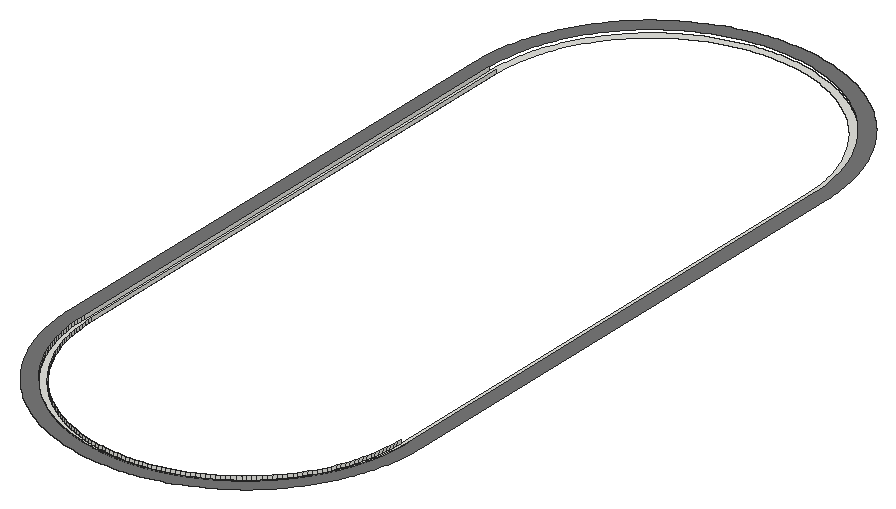
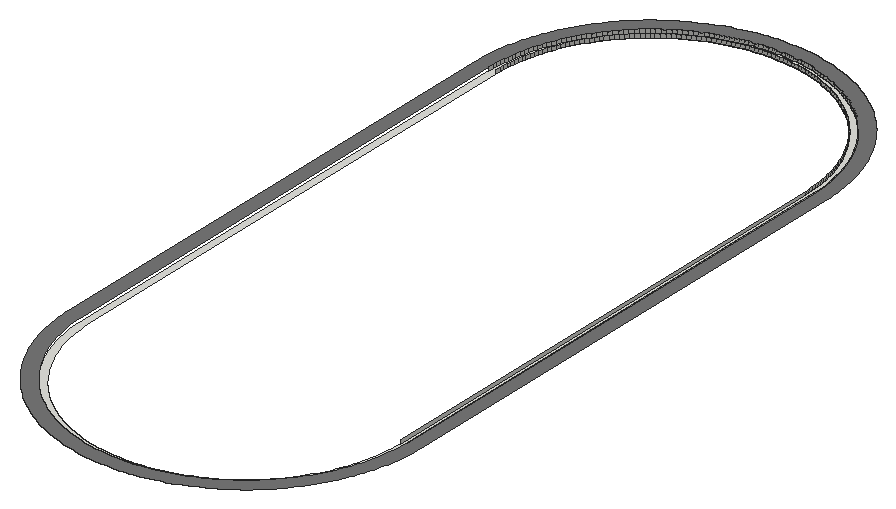
# SketchUp Ruby script. Lengths in inches.
U = 1.inch
M = Sketchup.active_model
def pt(a) = Geom::Point3d.new(a.map { |v| v * U })
def face(e, loops, mat)
  f = e.add_face(loops[0].map { |a| pt(a) })
  loops[1..].each { |l| e.add_face(l.map { |a| pt(a) }).erase! }
  f.material = f.back_material = mat if mat
  f
end
# faces: each face lists its corners as indices into pts; further lists are holes
def faces(e, pts, list, mat = nil) = list.each { |f| face(e, (f[0].is_a?(Array) ? f : [f]).map { |l| l.map { |i| pts[i] } }, mat) }
# xy, xz, yz: faces in a plane at the given z, y or x. An outline is a flat list of corners, or four numbers for a rectangle; further outlines are holes
def ring(l) = l.size == 4 ? [[l[0], l[1]], [l[2], l[1]], [l[2], l[3]], [l[0], l[3]]] : l.each_slice(2).to_a
def flat(e, list, mat, &to3) = list.each { |f| face(e, (f[0].is_a?(Array) ? f : [f]).map { |l| ring(l).map { |u, v| to3.(u, v) } }, mat) }
def xy(e, z, list, mat = nil) = flat(e, list, mat) { |x, y| [x, y, z] }
def xz(e, y, list, mat = nil) = flat(e, list, mat) { |x, z| [x, y, z] }
def yz(e, x, list, mat = nil) = flat(e, list, mat) { |y, z| [x, y, z] }
def lines(e, pts, list) = list.each { |a, b| e.add_line(pt(pts[a]), pt(pts[b])) }
# prism: a flat outline (further loops are holes) pulled along v
def prism(e, loops, v, mat = nil)
  f = face(e, loops, mat); d = Geom::Vector3d.new(v.map { |x| x * U })
  f.pushpull(f.normal.samedirection?(d) ? d.length : -d.length)
end
def box(e, o, s, mat = nil) = prism(e, [[o, [o[0] + s[0], o[1], o[2]], [o[0] + s[0], o[1] + s[1], o[2]], [o[0], o[1] + s[1], o[2]]]], [0, 0, s[2]], mat)
def at(x, y, z, deg = 0) = Geom::Transformation.translation(pt([x, y, z])) * Geom::Transformation.rotation(ORIGIN, Z_AXIS, deg.degrees)
def axes(o, x, y, z) = Geom::Transformation.new([*x, 0, *y, 0, *z, 0, *pt(o).to_a, 1])
def part(name) = M.definitions.add(name)
# library, detail: a bought-in or finely detailed component or shape, given as its bounding box
def library(name, o, s) = part(name).tap { |d| box(d.entities, o, s) }
def detail(e, o, s) = box(e.add_group.entities, o, s)
def put(e, d, t, mat = nil) = e.add_instance(d, t).tap { |i| i.material = mat if mat }
def group(e, t, mat = nil) = e.add_group.tap { |g| g.transformation = t; g.material = mat if mat }.entities
root = M.entities
M.materials.add("[Slate Light Tile]").color = [119, 119, 119]
xy(root,2.5,[[[189,25,189.6,25.01,190.2,25.03,190.8,25.07,191.4,25.125,192,25.2,192.6,25.28,193.78,25.5,194.37,25.64,194.95,25.78,195.53,25.95,196.11,26.125,196.68,26.32,197.24,26.53,197.8,26.75,198.35,26.99,198.9,27.24,199.44,27.51,199.97,27.79,200.5,28.08,201.02,28.39,201.53,28.71,202.03,29.05,202.52,29.39,203,29.75,203.47,30.125,203.9375,30.51,204.39,30.91,204.83,31.32,205.26,31.74,205.68,32.17,206.09,32.61,206.49,33.0625,206.875,33.53,207.25,34,207.61,34.48,207.95,34.97,208.29,35.47,208.61,35.98,208.92,36.5,209.21,37.03,209.49,37.56,209.76,38.1,210.01,38.65,210.25,39.2,210.47,39.76,210.68,40.32,210.875,40.89,211.05,41.47,211.22,42.05,211.36,42.63,211.5,43.22,211.72,44.4,211.8,45,211.875,45.6,211.93,46.2,211.97,46.8,211.99,47.4,212,48,212,120,211.99,120.6,211.97,121.2,211.93,121.8,211.875,122.4,211.8,123,211.72,123.6,211.5,124.78,211.36,125.37,211.22,125.95,211.05,126.53,210.875,127.11,210.68,127.68,210.47,128.24,210.25,128.8,210.01,129.35,209.76,129.9,209.49,130.44,209.21,130.97,208.92,131.5,208.61,132.02,208.29,132.53,207.95,133.03,207.61,133.52,207.25,134,206.875,134.47,206.49,134.9375,206.09,135.39,205.68,135.83,205.26,136.26,204.83,136.68,204.39,137.09,203.9375,137.49,203.47,137.875,203,138.25,202.52,138.61,202.03,138.95,201.53,139.29,201.02,139.61,200.5,139.92,199.97,140.21,199.44,140.49,198.9,140.76,198.35,141.01,197.8,141.25,197.24,141.47,196.68,141.68,196.11,141.875,195.53,142.05,194.95,142.22,194.37,142.36,193.78,142.5,192.6,142.72,192,142.8,191.4,142.875,190.8,142.93,190.2,142.97,189.6,142.99,189,143,188.4,142.99,187.8,142.97,187.2,142.93,186.6,142.875,186,142.8,185.4,142.72,184.22,142.5,183.63,142.36,183.05,142.22,182.47,142.05,181.89,141.875,181.32,141.68,180.76,141.47,180.2,141.25,179.65,141.01,179.1,140.76,178.56,140.49,178.03,140.21,177.5,139.92,176.98,139.61,176.47,139.29,175.97,138.95,175.48,138.61,175,138.25,174.53,137.875,174.0625,137.49,173.61,137.09,173.17,136.68,172.74,136.26,172.32,135.83,171.91,135.39,171.51,134.9375,171.125,134.47,170.75,134,170.39,133.52,170.05,133.03,169.71,132.53,169.39,132.02,169.08,131.5,168.79,130.97,168.51,130.44,168.24,129.9,167.99,129.35,167.75,128.8,167.53,128.24,167.32,127.68,167.125,127.11,166.95,126.53,166.78,125.95,166.64,125.37,166.5,124.78,166.28,123.6,166.2,123,166.125,122.4,166.07,121.8,166.03,121.2,166.01,120.6,166,120,166,48,166.01,47.4,166.03,46.8,166.07,46.2,166.125,45.6,166.2,45,166.28,44.4,166.5,43.22,166.64,42.63,166.78,42.05,166.95,41.47,167.125,40.89,167.32,40.32,167.53,39.76,167.75,39.2,167.99,38.65,168.24,38.1,168.51,37.56,168.79,37.03,169.08,36.5,169.39,35.98,169.71,35.47,170.05,34.97,170.39,34.48,170.75,34,171.125,33.53,171.51,33.0625,171.91,32.61,172.32,32.17,172.74,31.74,173.17,31.32,173.61,30.91,174.0625,30.51,174.53,30.125,175,29.75,175.48,29.39,175.97,29.05,176.47,28.71,176.98,28.39,177.5,28.08,178.03,27.79,178.56,27.51,179.1,27.24,179.65,26.99,180.2,26.75,180.76,26.53,181.32,26.32,181.89,26.125,182.47,25.95,183.05,25.78,183.63,25.64,184.22,25.5,185.4,25.28,186,25.2,186.6,25.125,187.2,25.07,187.8,25.03,188.4,25.01],[189,26,188.42,26.01,187.85,26.03,187.27,26.07,186.7,26.12,186.13,26.1875,185.56,26.27,184.99,26.37,184.43,26.48,183.86,26.61,183.31,26.75,182.75,26.91,182.2,27.08,181.66,27.26,181.12,27.46,180.58,27.67,180.05,27.9,179.53,28.14,179.01,28.4,178.5,28.67,178,28.95,177.51,29.24,177.02,29.55,176.54,29.87,176.07,30.2,175.15,30.9,174.71,31.27,174.28,31.65,173.86,32.04,173.44,32.44,173.04,32.86,172.65,33.28,172.27,33.71,171.9,34.15,171.2,35.07,170.87,35.54,170.55,36.02,170.24,36.51,169.95,37,169.67,37.5,169.4,38.01,169.14,38.53,168.9,39.05,168.67,39.58,168.46,40.12,168.26,40.66,168.08,41.2,167.91,41.75,167.75,42.31,167.61,42.86,167.48,43.43,167.37,43.99,167.27,44.56,167.1875,45.13,167.12,45.7,167.07,46.27,167.03,46.85,167.01,47.42,167,48,167,120,167.01,120.58,167.03,121.15,167.07,121.73,167.12,122.3,167.1875,122.87,167.27,123.44,167.37,124.01,167.48,124.57,167.61,125.14,167.75,125.69,167.91,126.25,168.08,126.8,168.26,127.34,168.46,127.88,168.67,128.42,168.9,128.95,169.14,129.47,169.4,129.99,169.67,130.5,169.95,131,170.24,131.49,170.55,131.98,170.87,132.46,171.2,132.93,171.9,133.85,172.27,134.29,172.65,134.72,173.04,135.14,173.44,135.56,173.86,135.96,174.28,136.35,174.71,136.73,175.15,137.1,176.07,137.8,176.54,138.13,177.02,138.45,177.51,138.76,178,139.05,178.5,139.33,179.01,139.6,179.53,139.86,180.05,140.1,180.58,140.33,181.12,140.54,181.66,140.74,182.2,140.92,182.75,141.09,183.31,141.25,183.86,141.39,184.43,141.52,184.99,141.63,185.56,141.73,186.13,141.8125,186.7,141.88,187.27,141.93,187.85,141.97,188.42,141.99,189,142,189.58,141.99,190.15,141.97,190.73,141.93,191.3,141.88,191.87,141.8125,192.44,141.73,193.01,141.63,193.57,141.52,194.14,141.39,194.69,141.25,195.25,141.09,195.8,140.92,196.34,140.74,196.88,140.54,197.42,140.33,197.95,140.1,198.47,139.86,198.99,139.6,199.5,139.33,200,139.05,200.49,138.76,200.98,138.45,201.46,138.13,201.93,137.8,202.85,137.1,203.29,136.73,203.72,136.35,204.14,135.96,204.56,135.56,204.96,135.14,205.35,134.72,205.73,134.29,206.1,133.85,206.8,132.93,207.13,132.46,207.45,131.98,207.76,131.49,208.05,131,208.33,130.5,208.6,129.99,208.86,129.47,209.1,128.95,209.33,128.42,209.54,127.88,209.74,127.34,209.92,126.8,210.09,126.25,210.25,125.69,210.39,125.14,210.52,124.57,210.63,124.01,210.73,123.44,210.8125,122.87,210.88,122.3,210.93,121.73,210.97,121.15,210.99,120.58,211,120,211,48,210.99,47.42,210.97,46.85,210.93,46.27,210.88,45.7,210.8125,45.13,210.73,44.56,210.63,43.99,210.52,43.43,210.39,42.86,210.25,42.31,210.09,41.75,209.92,41.2,209.74,40.66,209.54,40.12,209.33,39.58,209.1,39.05,208.86,38.53,208.6,38.01,208.33,37.5,208.05,37,207.76,36.51,207.45,36.02,207.13,35.54,206.8,35.07,206.1,34.15,205.73,33.71,205.35,33.28,204.96,32.86,204.56,32.44,204.14,32.04,203.72,31.65,203.29,31.27,202.85,30.9,201.93,30.2,201.46,29.87,200.98,29.55,200.49,29.24,200,28.95,199.5,28.67,198.99,28.4,198.47,28.14,197.95,27.9,197.42,27.67,196.88,27.46,196.34,27.26,195.8,27.08,195.25,26.91,194.69,26.75,194.14,26.61,193.57,26.48,193.01,26.37,192.44,26.27,191.87,26.1875,191.3,26.12,190.73,26.07,190.15,26.03,189.58,26.01]]])
xy(root,3,[[[189,23,189.65,23.01,190.31,23.03,190.96,23.08,191.61,23.14,192.26,23.21,192.91,23.31,193.56,23.42,194.2,23.55,194.84,23.69,195.47,23.85,196.1,24.03,196.73,24.22,197.35,24.43,197.96,24.66,198.57,24.9,199.17,25.16,200.35,25.72,200.93,26.03,201.5,26.35,202.0625,26.68,202.62,27.03,203.16,27.4,203.69,27.77,204.22,28.17,204.73,28.57,205.24,28.99,205.73,29.42,206.21,29.87,206.68,30.32,207.13,30.79,207.58,31.27,208.01,31.76,208.43,32.27,208.83,32.78,209.23,33.31,209.6,33.84,209.97,34.38,210.32,34.9375,210.65,35.5,210.97,36.07,211.28,36.65,211.84,37.83,212.1,38.43,212.34,39.04,212.57,39.65,212.78,40.27,212.97,40.9,213.15,41.53,213.31,42.16,213.45,42.8,213.58,43.44,213.69,44.09,213.79,44.74,213.86,45.39,213.92,46.04,213.97,46.69,213.99,47.35,214,48,214,120,213.99,120.65,213.97,121.31,213.92,121.96,213.86,122.61,213.79,123.26,213.69,123.91,213.58,124.56,213.45,125.2,213.31,125.84,213.15,126.47,212.97,127.1,212.78,127.73,212.57,128.35,212.34,128.96,212.1,129.57,211.84,130.17,211.28,131.35,210.97,131.93,210.65,132.5,210.32,133.0625,209.97,133.62,209.6,134.16,209.23,134.69,208.83,135.22,208.43,135.73,208.01,136.24,207.58,136.73,207.13,137.21,206.68,137.68,206.21,138.13,205.73,138.58,205.24,139.01,204.73,139.43,204.22,139.83,203.69,140.23,203.16,140.6,202.62,140.97,202.0625,141.32,201.5,141.65,200.93,141.97,200.35,142.28,199.17,142.84,198.57,143.1,197.96,143.34,197.35,143.57,196.73,143.78,196.1,143.97,195.47,144.15,194.84,144.31,194.2,144.45,193.56,144.58,192.91,144.69,192.26,144.79,191.61,144.86,190.96,144.92,190.31,144.97,189.65,144.99,189,145,188.35,144.99,187.69,144.97,187.04,144.92,186.39,144.86,185.74,144.79,185.09,144.69,184.44,144.58,183.8,144.45,183.16,144.31,182.53,144.15,181.9,143.97,181.27,143.78,180.65,143.57,180.04,143.34,179.43,143.1,178.83,142.84,177.65,142.28,177.07,141.97,176.5,141.65,175.9375,141.32,175.38,140.97,174.84,140.6,174.31,140.23,173.78,139.83,173.27,139.43,172.76,139.01,172.27,138.58,171.79,138.13,171.32,137.68,170.87,137.21,170.42,136.73,169.99,136.24,169.57,135.73,169.17,135.22,168.77,134.69,168.4,134.16,168.03,133.62,167.68,133.0625,167.35,132.5,167.03,131.93,166.72,131.35,166.16,130.17,165.9,129.57,165.66,128.96,165.43,128.35,165.22,127.73,165.03,127.1,164.85,126.47,164.69,125.84,164.55,125.2,164.42,124.56,164.31,123.91,164.21,123.26,164.14,122.61,164.08,121.96,164.03,121.31,164.01,120.65,164,120,164,48,164.01,47.35,164.03,46.69,164.08,46.04,164.14,45.39,164.21,44.74,164.31,44.09,164.42,43.44,164.55,42.8,164.69,42.16,164.85,41.53,165.03,40.9,165.22,40.27,165.43,39.65,165.66,39.04,165.9,38.43,166.16,37.83,166.72,36.65,167.03,36.07,167.35,35.5,167.68,34.9375,168.03,34.38,168.4,33.84,168.77,33.31,169.17,32.78,169.57,32.27,169.99,31.76,170.42,31.27,170.87,30.79,171.32,30.32,171.79,29.87,172.27,29.42,172.76,28.99,173.27,28.57,173.78,28.17,174.31,27.77,174.84,27.4,175.38,27.03,175.9375,26.68,176.5,26.35,177.07,26.03,177.65,25.72,178.83,25.16,179.43,24.9,180.04,24.66,180.65,24.43,181.27,24.22,181.9,24.03,182.53,23.85,183.16,23.69,183.8,23.55,184.44,23.42,185.09,23.31,185.74,23.21,186.39,23.14,187.04,23.08,187.69,23.03,188.35,23.01],[189,25,188.4,25.01,187.8,25.03,187.2,25.07,186.6,25.125,186,25.2,185.4,25.28,184.22,25.5,183.63,25.64,183.05,25.78,182.47,25.95,181.89,26.125,181.32,26.32,180.76,26.53,180.2,26.75,179.65,26.99,179.1,27.24,178.56,27.51,178.03,27.79,177.5,28.08,176.98,28.39,176.47,28.71,175.97,29.05,175.48,29.39,175,29.75,174.53,30.125,174.0625,30.51,173.61,30.91,173.17,31.32,172.74,31.74,172.32,32.17,171.91,32.61,171.51,33.0625,171.125,33.53,170.75,34,170.39,34.48,170.05,34.97,169.71,35.47,169.39,35.98,169.08,36.5,168.79,37.03,168.51,37.56,168.24,38.1,167.99,38.65,167.75,39.2,167.53,39.76,167.32,40.32,167.125,40.89,166.95,41.47,166.78,42.05,166.64,42.63,166.5,43.22,166.28,44.4,166.2,45,166.125,45.6,166.07,46.2,166.03,46.8,166.01,47.4,166,48,166,120,166.01,120.6,166.03,121.2,166.07,121.8,166.125,122.4,166.2,123,166.28,123.6,166.5,124.78,166.64,125.37,166.78,125.95,166.95,126.53,167.125,127.11,167.32,127.68,167.53,128.24,167.75,128.8,167.99,129.35,168.24,129.9,168.51,130.44,168.79,130.97,169.08,131.5,169.39,132.02,169.71,132.53,170.05,133.03,170.39,133.52,170.75,134,171.125,134.47,171.51,134.9375,171.91,135.39,172.32,135.83,172.74,136.26,173.17,136.68,173.61,137.09,174.0625,137.49,174.53,137.875,175,138.25,175.48,138.61,175.97,138.95,176.47,139.29,176.98,139.61,177.5,139.92,178.03,140.21,178.56,140.49,179.1,140.76,179.65,141.01,180.2,141.25,180.76,141.47,181.32,141.68,181.89,141.875,182.47,142.05,183.05,142.22,183.63,142.36,184.22,142.5,185.4,142.72,186,142.8,186.6,142.875,187.2,142.93,187.8,142.97,188.4,142.99,189,143,189.6,142.99,190.2,142.97,190.8,142.93,191.4,142.875,192,142.8,192.6,142.72,193.78,142.5,194.37,142.36,194.95,142.22,195.53,142.05,196.11,141.875,196.68,141.68,197.24,141.47,197.8,141.25,198.35,141.01,198.9,140.76,199.44,140.49,199.97,140.21,200.5,139.92,201.02,139.61,201.53,139.29,202.03,138.95,202.52,138.61,203,138.25,203.47,137.875,203.9375,137.49,204.39,137.09,204.83,136.68,205.26,136.26,205.68,135.83,206.09,135.39,206.49,134.9375,206.875,134.47,207.25,134,207.61,133.52,207.95,133.03,208.29,132.53,208.61,132.02,208.92,131.5,209.21,130.97,209.49,130.44,209.76,129.9,210.01,129.35,210.25,128.8,210.47,128.24,210.68,127.68,210.875,127.11,211.05,126.53,211.22,125.95,211.36,125.37,211.5,124.78,211.72,123.6,211.8,123,211.875,122.4,211.93,121.8,211.97,121.2,211.99,120.6,212,120,212,48,211.99,47.4,211.97,46.8,211.93,46.2,211.875,45.6,211.8,45,211.72,44.4,211.5,43.22,211.36,42.63,211.22,42.05,211.05,41.47,210.875,40.89,210.68,40.32,210.47,39.76,210.25,39.2,210.01,38.65,209.76,38.1,209.49,37.56,209.21,37.03,208.92,36.5,208.61,35.98,208.29,35.47,207.95,34.97,207.61,34.48,207.25,34,206.875,33.53,206.49,33.0625,206.09,32.61,205.68,32.17,205.26,31.74,204.83,31.32,204.39,30.91,203.9375,30.51,203.47,30.125,203,29.75,202.52,29.39,202.03,29.05,201.53,28.71,201.02,28.39,200.5,28.08,199.97,27.79,199.44,27.51,198.9,27.24,198.35,26.99,197.8,26.75,197.24,26.53,196.68,26.32,196.11,26.125,195.53,25.95,194.95,25.78,194.37,25.64,193.78,25.5,192.6,25.28,192,25.2,191.4,25.125,190.8,25.07,190.2,25.03,189.6,25.01]]],"[Slate Light Tile]")
yz(root,166,[[48,2.5,120,3]])
yz(root,167,[[48,2.5,120,3]])
p = [[187.2,25.07,3],[187.8,25.03,3],[187.8,25.03,2.5],[187.2,25.07,2.5],[188.4,25.01,3],[188.4,25.01,2.5],
  [189,25,3],[189,25,2.5],[189.6,25.01,3],[189.6,25.01,2.5],[190.2,25.03,3],[190.2,25.03,2.5],
  [190.8,25.07,3],[190.8,25.07,2.5],[186,25.2,3],[186.6,25.125,3],[186.6,25.125,2.5],[186,25.2,2.5],
  [191.4,25.125,3],[191.4,25.125,2.5],[192,25.2,3],[192,25.2,2.5],[185.4,25.28,3],[185.4,25.28,2.5],
  [192.6,25.28,3],[192.6,25.28,2.5],[184.81,25.39,3],[184.81,25.39,2.5],[193.19,25.39,3],[193.19,25.39,2.5],
  [184.22,25.5,3],[184.22,25.5,2.5],[193.78,25.5,3],[193.78,25.5,2.5],[183.63,25.64,3],[183.63,25.64,2.5],
  [194.37,25.64,3],[194.37,25.64,2.5],[183.05,25.78,3],[183.05,25.78,2.5],[194.95,25.78,3],[194.95,25.78,2.5],
  [182.47,25.95,3],[182.47,25.95,2.5],[195.53,25.95,3],[195.53,25.95,2.5],[181.89,26.125,3],[181.89,26.125,2.5],
  [196.11,26.125,3],[196.11,26.125,2.5],[187.85,26.03,3],[187.27,26.07,3],[187.27,26.07,2.5],[187.85,26.03,2.5],
  [188.42,26.01,3],[188.42,26.01,2.5],[189,26,3],[189,26,2.5],[189.58,26.01,3],[189.58,26.01,2.5],
  [190.15,26.03,3],[190.15,26.03,2.5],[190.73,26.07,3],[190.73,26.07,2.5],[181.32,26.32,3],[181.32,26.32,2.5],
  [186.7,26.12,3],[186.13,26.1875,3],[186.13,26.1875,2.5],[186.7,26.12,2.5],[191.3,26.12,3],[191.3,26.12,2.5],
  [191.87,26.1875,3],[191.87,26.1875,2.5],[196.68,26.32,3],[196.68,26.32,2.5],[185.56,26.27,3],[185.56,26.27,2.5],
  [192.44,26.27,3],[192.44,26.27,2.5],[180.76,26.53,3],[180.76,26.53,2.5],[184.99,26.37,3],[184.99,26.37,2.5],
  [193.01,26.37,3],[193.01,26.37,2.5],[197.24,26.53,3],[197.24,26.53,2.5],[184.43,26.48,3],[184.43,26.48,2.5],
  [193.57,26.48,3],[193.57,26.48,2.5],[180.2,26.75,3],[180.2,26.75,2.5],[183.86,26.61,3],[183.86,26.61,2.5],
  [194.14,26.61,3],[194.14,26.61,2.5],[197.8,26.75,3],[197.8,26.75,2.5],[183.31,26.75,3],[183.31,26.75,2.5],
  [194.69,26.75,3],[194.69,26.75,2.5],[182.75,26.91,3],[182.75,26.91,2.5],[195.25,26.91,3],[195.25,26.91,2.5],
  [179.65,26.99,3],[179.65,26.99,2.5],[198.35,26.99,3],[198.35,26.99,2.5],[182.2,27.08,3],[182.2,27.08,2.5],
  [195.8,27.08,3],[195.8,27.08,2.5],[179.1,27.24,3],[179.1,27.24,2.5],[198.9,27.24,3],[198.9,27.24,2.5],
  [181.66,27.26,3],[181.66,27.26,2.5],[196.34,27.26,3],[196.34,27.26,2.5],[178.56,27.51,3],[178.56,27.51,2.5],
  [199.44,27.51,3],[199.44,27.51,2.5],[181.12,27.46,3],[181.12,27.46,2.5],[196.88,27.46,3],[196.88,27.46,2.5],
  [178.03,27.79,3],[178.03,27.79,2.5],[180.58,27.67,3],[180.58,27.67,2.5],[197.42,27.67,3],[197.42,27.67,2.5],
  [199.97,27.79,3],[199.97,27.79,2.5],[180.05,27.9,3],[180.05,27.9,2.5],[197.95,27.9,3],[197.95,27.9,2.5],
  [177.5,28.08,3],[177.5,28.08,2.5],[200.5,28.08,3],[200.5,28.08,2.5],[179.53,28.14,3],[179.53,28.14,2.5],
  [198.47,28.14,3],[198.47,28.14,2.5],[176.98,28.39,3],[176.98,28.39,2.5],[179.01,28.4,3],[179.01,28.4,2.5],
  [198.99,28.4,3],[198.99,28.4,2.5],[201.02,28.39,3],[201.02,28.39,2.5],[176.47,28.71,3],[176.47,28.71,2.5],
  [178.5,28.67,3],[178.5,28.67,2.5],[199.5,28.67,3],[199.5,28.67,2.5],[201.53,28.71,3],[201.53,28.71,2.5],
  [175.97,29.05,3],[175.97,29.05,2.5],[178,28.95,3],[178,28.95,2.5],[200,28.95,3],[200,28.95,2.5],
  [202.03,29.05,3],[202.03,29.05,2.5],[177.51,29.24,3],[177.51,29.24,2.5],[200.49,29.24,3],[200.49,29.24,2.5],
  [175.48,29.39,3],[175.48,29.39,2.5],[202.52,29.39,3],[202.52,29.39,2.5],[177.02,29.55,3],[177.02,29.55,2.5],
  [200.98,29.55,3],[200.98,29.55,2.5],[175,29.75,3],[175,29.75,2.5],[203,29.75,3],[203,29.75,2.5],
  [176.54,29.87,3],[176.54,29.87,2.5],[201.46,29.87,3],[201.46,29.87,2.5],[174.53,30.125,3],[174.53,30.125,2.5],
  [203.47,30.125,3],[203.47,30.125,2.5],[176.07,30.2,3],[176.07,30.2,2.5],[201.93,30.2,3],[201.93,30.2,2.5],
  [174.0625,30.51,3],[174.0625,30.51,2.5],[203.9375,30.51,3],[203.9375,30.51,2.5],[175.61,30.55,3],[175.61,30.55,2.5],
  [202.39,30.55,3],[202.39,30.55,2.5],[173.61,30.91,3],[173.61,30.91,2.5],[175.15,30.9,3],[175.15,30.9,2.5],
  [202.85,30.9,3],[202.85,30.9,2.5],[204.39,30.91,3],[204.39,30.91,2.5],[173.17,31.32,3],[173.17,31.32,2.5],
  [174.71,31.27,3],[174.71,31.27,2.5],[203.29,31.27,3],[203.29,31.27,2.5],[204.83,31.32,3],[204.83,31.32,2.5],
  [172.74,31.74,3],[172.74,31.74,2.5],[174.28,31.65,3],[174.28,31.65,2.5],[203.72,31.65,3],[203.72,31.65,2.5],
  [205.26,31.74,3],[205.26,31.74,2.5],[172.32,32.17,3],[172.32,32.17,2.5],[173.86,32.04,3],[173.86,32.04,2.5],
  [204.14,32.04,3],[204.14,32.04,2.5],[205.68,32.17,3],[205.68,32.17,2.5],[173.44,32.44,3],[173.44,32.44,2.5],
  [204.56,32.44,3],[204.56,32.44,2.5],[171.91,32.61,3],[171.91,32.61,2.5],[206.09,32.61,3],[206.09,32.61,2.5],
  [173.04,32.86,3],[173.04,32.86,2.5],[204.96,32.86,3],[204.96,32.86,2.5],[171.51,33.0625,3],[171.51,33.0625,2.5],
  [206.49,33.0625,3],[206.49,33.0625,2.5],[172.65,33.28,3],[172.65,33.28,2.5],[205.35,33.28,3],[205.35,33.28,2.5],
  [171.125,33.53,3],[171.125,33.53,2.5],[206.875,33.53,3],[206.875,33.53,2.5],[172.27,33.71,3],[172.27,33.71,2.5],
  [205.73,33.71,3],[205.73,33.71,2.5],[170.75,34,3],[170.75,34,2.5],[207.25,34,3],[207.25,34,2.5],
  [171.9,34.15,3],[171.9,34.15,2.5],[206.1,34.15,3],[206.1,34.15,2.5],[170.39,34.48,3],[170.39,34.48,2.5],
  [207.61,34.48,3],[207.61,34.48,2.5],[171.55,34.61,3],[171.55,34.61,2.5],[206.45,34.61,3],[206.45,34.61,2.5],
  [170.05,34.97,3],[170.05,34.97,2.5],[207.95,34.97,3],[207.95,34.97,2.5],[171.2,35.07,3],[171.2,35.07,2.5],
  [206.8,35.07,3],[206.8,35.07,2.5],[169.71,35.47,3],[169.71,35.47,2.5],[208.29,35.47,3],[208.29,35.47,2.5],
  [170.87,35.54,3],[170.87,35.54,2.5],[207.13,35.54,3],[207.13,35.54,2.5],[169.39,35.98,3],[169.39,35.98,2.5],
  [170.55,36.02,3],[170.55,36.02,2.5],[207.45,36.02,3],[207.45,36.02,2.5],[208.61,35.98,3],[208.61,35.98,2.5],
  [169.08,36.5,3],[169.08,36.5,2.5],[170.24,36.51,3],[170.24,36.51,2.5],[207.76,36.51,3],[207.76,36.51,2.5],
  [208.92,36.5,3],[208.92,36.5,2.5],[168.79,37.03,3],[168.79,37.03,2.5],[169.95,37,3],[169.95,37,2.5],
  [208.05,37,3],[208.05,37,2.5],[209.21,37.03,3],[209.21,37.03,2.5],[168.51,37.56,3],[168.51,37.56,2.5],
  [169.67,37.5,3],[169.67,37.5,2.5],[208.33,37.5,3],[208.33,37.5,2.5],[209.49,37.56,3],[209.49,37.56,2.5],
  [169.4,38.01,3],[169.4,38.01,2.5],[208.6,38.01,3],[208.6,38.01,2.5],[168.24,38.1,3],[168.24,38.1,2.5],
  [209.76,38.1,3],[209.76,38.1,2.5],[169.14,38.53,3],[169.14,38.53,2.5],[208.86,38.53,3],[208.86,38.53,2.5],
  [167.99,38.65,3],[167.99,38.65,2.5],[210.01,38.65,3],[210.01,38.65,2.5],[168.9,39.05,3],[168.9,39.05,2.5],
  [209.1,39.05,3],[209.1,39.05,2.5],[167.75,39.2,3],[167.75,39.2,2.5],[210.25,39.2,3],[210.25,39.2,2.5],
  [168.67,39.58,3],[168.67,39.58,2.5],[209.33,39.58,3],[209.33,39.58,2.5],[167.53,39.76,3],[167.53,39.76,2.5],
  [210.47,39.76,3],[210.47,39.76,2.5],[168.46,40.12,3],[168.46,40.12,2.5],[209.54,40.12,3],[209.54,40.12,2.5],
  [167.32,40.32,3],[167.32,40.32,2.5],[210.68,40.32,3],[210.68,40.32,2.5],[168.26,40.66,3],[168.26,40.66,2.5],
  [209.74,40.66,3],[209.74,40.66,2.5],[167.125,40.89,3],[167.125,40.89,2.5],[210.875,40.89,3],[210.875,40.89,2.5],
  [168.08,41.2,3],[168.08,41.2,2.5],[209.92,41.2,3],[209.92,41.2,2.5],[166.95,41.47,3],[166.95,41.47,2.5],
  [211.05,41.47,3],[211.05,41.47,2.5],[167.91,41.75,3],[167.91,41.75,2.5],[210.09,41.75,3],[210.09,41.75,2.5],
  [166.78,42.05,3],[166.78,42.05,2.5],[211.22,42.05,3],[211.22,42.05,2.5],[167.75,42.31,3],[167.75,42.31,2.5],
  [210.25,42.31,3],[210.25,42.31,2.5],[166.64,42.63,3],[166.64,42.63,2.5],[211.36,42.63,3],[211.36,42.63,2.5],
  [167.61,42.86,3],[167.61,42.86,2.5],[210.39,42.86,3],[210.39,42.86,2.5],[166.5,43.22,3],[166.5,43.22,2.5],
  [211.5,43.22,3],[211.5,43.22,2.5],[167.48,43.43,3],[167.48,43.43,2.5],[210.52,43.43,3],[210.52,43.43,2.5],
  [166.39,43.81,3],[166.39,43.81,2.5],[211.61,43.81,3],[211.61,43.81,2.5],[167.37,43.99,3],[167.37,43.99,2.5],
  [210.63,43.99,3],[210.63,43.99,2.5],[166.28,44.4,3],[166.28,44.4,2.5],[211.72,44.4,3],[211.72,44.4,2.5],
  [167.27,44.56,3],[167.27,44.56,2.5],[210.73,44.56,3],[210.73,44.56,2.5],[166.2,45,3],[166.2,45,2.5],
  [211.8,45,3],[211.8,45,2.5],[167.1875,45.13,3],[167.1875,45.13,2.5],[210.8125,45.13,3],[210.8125,45.13,2.5],
  [166.125,45.6,3],[166.125,45.6,2.5],[211.875,45.6,3],[211.875,45.6,2.5],[167.12,45.7,3],[167.12,45.7,2.5],
  [210.88,45.7,3],[210.88,45.7,2.5],[166.07,46.2,3],[166.07,46.2,2.5],[211.93,46.2,3],[211.93,46.2,2.5],
  [167.07,46.27,3],[167.07,46.27,2.5],[210.93,46.27,3],[210.93,46.27,2.5],[166.03,46.8,3],[166.03,46.8,2.5],
  [211.97,46.8,3],[211.97,46.8,2.5],[167.03,46.85,3],[167.03,46.85,2.5],[210.97,46.85,3],[210.97,46.85,2.5],
  [166.01,47.4,3],[166.01,47.4,2.5],[167.01,47.42,3],[167.01,47.42,2.5],[210.99,47.42,3],[210.99,47.42,2.5],
  [211.99,47.4,3],[211.99,47.4,2.5],[166,48,3],[166,48,2.5],[167,48,3],[167,48,2.5],
  [211,48,3],[211,48,2.5],[212,48,3],[212,48,2.5]]
faces(root,p,[[0,1,2,3],[1,4,5,2],[4,6,7,5],[6,8,9,7],[8,10,11,9],[10,12,13,11],[14,15,16,17],[15,0,3,16],
  [12,18,19,13],[18,20,21,19],[22,14,17,23],[20,24,25,21],[26,22,23,27],[24,28,29,25],[30,26,27,31],[28,32,33,29],
  [34,30,31,35],[32,36,37,33],[38,34,35,39],[36,40,41,37],[42,38,39,43],[40,44,45,41],[46,42,43,47],[44,48,49,45],
  [50,51,52,53],[54,50,53,55],[56,54,55,57],[58,56,57,59],[60,58,59,61],[62,60,61,63],[64,46,47,65],[66,67,68,69],
  [51,66,69,52],[70,62,63,71],[72,70,71,73],[48,74,75,49],[67,76,77,68],[78,72,73,79],[80,64,65,81],[76,82,83,77],
  [84,78,79,85],[74,86,87,75],[82,88,89,83],[90,84,85,91],[92,80,81,93],[88,94,95,89],[96,90,91,97],[86,98,99,87],
  [94,100,101,95],[102,96,97,103],[100,104,105,101],[106,102,103,107],[108,92,93,109],[98,110,111,99],[104,112,113,105],[114,106,107,115],
  [116,108,109,117],[110,118,119,111],[112,120,121,113],[122,114,115,123],[124,116,117,125],[118,126,127,119],[120,128,129,121],[130,122,123,131],
  [132,124,125,133],[128,134,135,129],[136,130,131,137],[126,138,139,127],[134,140,141,135],[142,136,137,143],[144,132,133,145],[138,146,147,139],
  [140,148,149,141],[150,142,143,151],[152,144,145,153],[148,154,155,149],[156,150,151,157],[146,158,159,147],[160,152,153,161],[154,162,163,155],
  [164,156,157,165],[158,166,167,159],[168,160,161,169],[162,170,171,163],[172,164,165,173],[166,174,175,167],[170,176,177,171],[178,172,173,179],
  [180,168,169,181],[174,182,183,175],[176,184,185,177],[186,178,179,187],[188,180,181,189],[182,190,191,183],[184,192,193,185],[194,186,187,195],
  [196,188,189,197],[190,198,199,191],[192,200,201,193],[202,194,195,203],[204,196,197,205],[198,206,207,199],[200,208,209,201],[210,202,203,211],
  [212,204,205,213],[208,214,215,209],[216,210,211,217],[206,218,219,207],[220,212,213,221],[214,222,223,215],[224,216,217,225],[218,226,227,219],
  [228,220,221,229],[222,230,231,223],[232,224,225,233],[226,234,235,227],[236,228,229,237],[230,238,239,231],[240,232,233,241],[234,242,243,235],
  [238,244,245,239],[246,240,241,247],[248,236,237,249],[242,250,251,243],[244,252,253,245],[254,246,247,255],[256,248,249,257],[250,258,259,251],
  [252,260,261,253],[262,254,255,263],[264,256,257,265],[258,266,267,259],[260,268,269,261],[270,262,263,271],[272,264,265,273],[266,274,275,267],
  [268,276,277,269],[278,270,271,279],[280,272,273,281],[274,282,283,275],[276,284,285,277],[286,278,279,287],[288,280,281,289],[282,290,291,283],
  [284,292,293,285],[294,286,287,295],[296,288,289,297],[290,298,299,291],[292,300,301,293],[302,294,295,303],[304,296,297,305],[300,306,307,301],
  [308,302,303,309],[298,310,311,299],[312,304,305,313],[306,314,315,307],[316,308,309,317],[310,318,319,311],[320,312,313,321],[314,322,323,315],
  [324,316,317,325],[318,326,327,319],[328,320,321,329],[322,330,331,323],[332,324,325,333],[326,334,335,327],[330,336,337,331],[338,332,333,339],
  [340,328,329,341],[334,342,343,335],[336,344,345,337],[346,338,339,347],[348,340,341,349],[342,350,351,343],[344,352,353,345],[354,346,347,355],
  [356,348,349,357],[350,358,359,351],[352,360,361,353],[362,354,355,363],[364,356,357,365],[358,366,367,359],[360,368,369,361],[370,362,363,371],
  [372,364,365,373],[366,374,375,367],[368,376,377,369],[378,370,371,379],[380,372,373,381],[374,382,383,375],[376,384,385,377],[386,378,379,387],
  [388,380,381,389],[382,390,391,383],[384,392,393,385],[394,386,387,395],[396,388,389,397],[390,398,399,391],[392,400,401,393],[402,394,395,403],
  [404,396,397,405],[398,406,407,399],[400,408,409,401],[410,402,403,411],[412,404,405,413],[406,414,415,407],[408,416,417,409],[418,410,411,419],
  [420,412,413,421],[414,422,423,415],[416,424,425,417],[426,418,419,427],[428,420,421,429],[422,430,431,423],[424,432,433,425],[434,426,427,435],
  [436,428,429,437],[430,438,439,431],[432,440,441,433],[442,434,435,443],[444,436,437,445],[438,446,447,439],[440,448,449,441],[450,442,443,451],
  [452,444,445,453],[446,454,455,447],[448,456,457,449],[458,450,451,459],[460,452,453,461],[454,462,463,455],[456,464,465,457],[466,458,459,467],
  [468,460,461,469],[464,470,471,465],[472,466,467,473],[462,474,475,463],[476,468,469,477],[470,478,479,471],[480,472,473,481],[474,482,483,475]])
